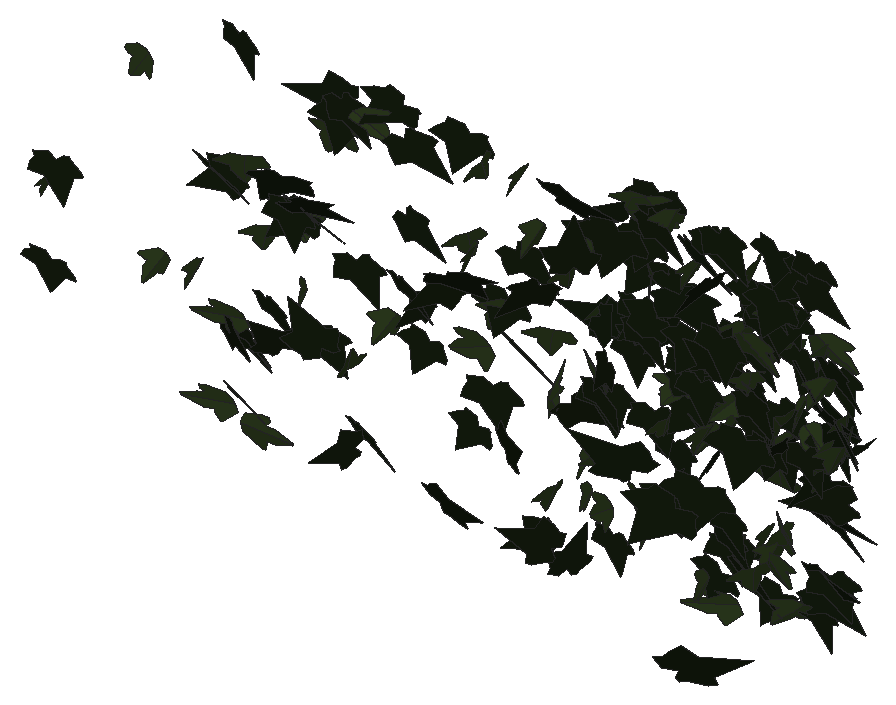
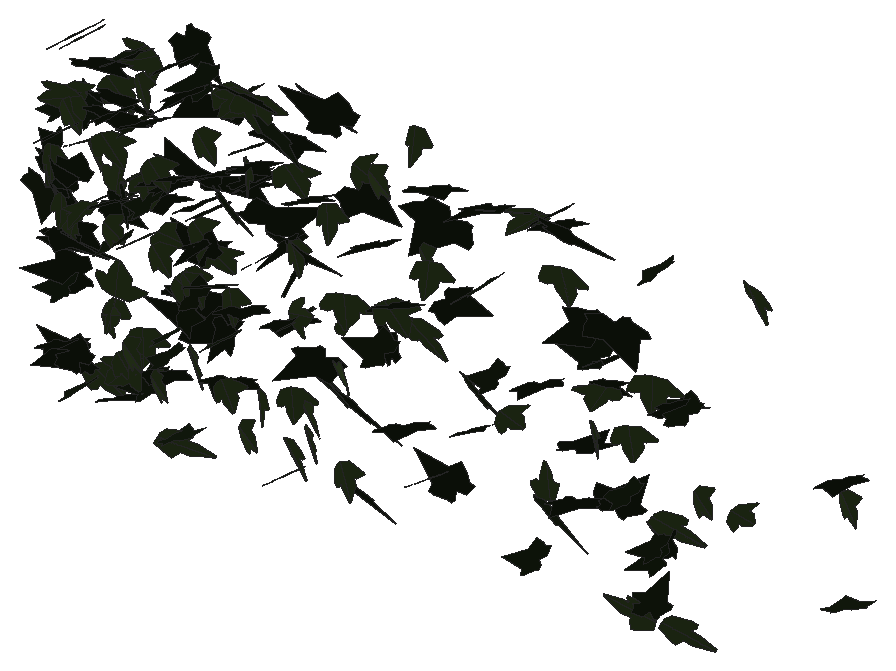
# SketchUp Ruby script. Lengths in millimetres.
U = 1.mm
M = Sketchup.active_model
def pt(a) = Geom::Point3d.new(a.map { |v| v * U })
def face(e, loops, mat)
  f = e.add_face(loops[0].map { |a| pt(a) })
  loops[1..].each { |l| e.add_face(l.map { |a| pt(a) }).erase! }
  f.material = f.back_material = mat if mat
  f
end
# faces: each face lists its corners as indices into pts; further lists are holes
def faces(e, pts, list, mat = nil) = list.each { |f| face(e, (f[0].is_a?(Array) ? f : [f]).map { |l| l.map { |i| pts[i] } }, mat) }
# xy, xz, yz: faces in a plane at the given z, y or x. An outline is a flat list of corners, or four numbers for a rectangle; further outlines are holes
def ring(l) = l.size == 4 ? [[l[0], l[1]], [l[2], l[1]], [l[2], l[3]], [l[0], l[3]]] : l.each_slice(2).to_a
def flat(e, list, mat, &to3) = list.each { |f| face(e, (f[0].is_a?(Array) ? f : [f]).map { |l| ring(l).map { |u, v| to3.(u, v) } }, mat) }
def xy(e, z, list, mat = nil) = flat(e, list, mat) { |x, y| [x, y, z] }
def xz(e, y, list, mat = nil) = flat(e, list, mat) { |x, z| [x, y, z] }
def yz(e, x, list, mat = nil) = flat(e, list, mat) { |y, z| [x, y, z] }
def lines(e, pts, list) = list.each { |a, b| e.add_line(pt(pts[a]), pt(pts[b])) }
# prism: a flat outline (further loops are holes) pulled along v
def prism(e, loops, v, mat = nil)
  f = face(e, loops, mat); d = Geom::Vector3d.new(v.map { |x| x * U })
  f.pushpull(f.normal.samedirection?(d) ? d.length : -d.length)
end
def box(e, o, s, mat = nil) = prism(e, [[o, [o[0] + s[0], o[1], o[2]], [o[0] + s[0], o[1] + s[1], o[2]], [o[0], o[1] + s[1], o[2]]]], [0, 0, s[2]], mat)
def at(x, y, z, deg = 0) = Geom::Transformation.translation(pt([x, y, z])) * Geom::Transformation.rotation(ORIGIN, Z_AXIS, deg.degrees)
def axes(o, x, y, z) = Geom::Transformation.new([*x, 0, *y, 0, *z, 0, *pt(o).to_a, 1])
def part(name) = M.definitions.add(name)
# library, detail: a bought-in or finely detailed component or shape, given as its bounding box
def library(name, o, s) = part(name).tap { |d| box(d.entities, o, s) }
def detail(e, o, s) = box(e.add_group.entities, o, s)
def put(e, d, t, mat = nil) = e.add_instance(d, t).tap { |i| i.material = mat if mat }
def group(e, t, mat = nil) = e.add_group.tap { |g| g.transformation = t; g.material = mat if mat }.entities
root = M.entities
M.materials.add("efeu1").color = [18, 25, 13]
M.materials.add("efeu2").color = [43, 57, 29]
c1 = part("ivyleaf_9")
p = [[39.1,54.8,31.7],[34.5,51.8,30.2],[-5.3,25.2,17.3],[-17.9,28.3,20.9],[-21.6,21.7,17],[-20.2,4.3,5.3],
  [-22.9,-0.3,2.5],[-17.1,-4,-0.6],[-2,-2.1,-1.2],[-0.7,-15.4,-10.1],[16.6,-22.3,-16.7],[21.1,-15.1,-12.5],
  [32.7,-10.7,-11],[46.1,-1.8,-6.6],[30.8,11.2,3.8]]
faces(c1.entities,p,[[0,1,2,3,4,5,6,7,8,9,10,11,12,13,14]],"efeu1")
c2 = part("ivyleaf_10")
p = [[0,12.8,-0.8],[-1.5,51.3,-10.9],[-4.9,51,-11.6],[-13.6,26.5,-7.3],[-13.2,15.9,-4.6],[-21.1,19.3,-7.2],
  [-29.5,16.3,-8.3],[-29.2,8.3,-6.2],[-19.7,-9.8,0.5],[-7.6,-13,4],[1,-12.2,5.8],[-0.4,51.1,-11.1],
  [-1.5,51.1,-10.9],[1,-12.4,5.9],[16.9,-12.4,3.5],[35.1,9.1,-5.1],[35,12.9,-6.1],[20.5,16.4,-4.9],
  [15.8,15,-3.8],[15.3,27.6,-7.1],[12.8,31.3,-7.8]]
faces(c2.entities,p,[[0,1,2,3,4,5,6,7,8,9,10],[11,12,0,13,14,15,16,17,18,19,20]],"efeu2")
put(root,c1,axes([1191.5,726.7,2811.6],[-0.73704,-0.9227,0.38725],[0.48551,-0.49255,-0.91849],[1.84155,-0.23943,0.39714]))
put(root,c2,axes([1219.3,690.7,3035.7],[0.12928,-1.10361,0.0718],[0.0069,-0.07171,-1.1057],[2.10482,0.06802,-0.00078]))
put(root,c1,axes([1236.5,686.2,3073.2],[-0.46682,-1.0606,-0.23525],[0.05512,0.2347,-1.08833],[2.06686,-0.24581,-0.02411]))
put(root,c2,axes([1480.5,663.3,3412.6],[1.55234,-0.77415,-0.31621],[-0.3436,0.26829,-1.1225],[1.55401,0.83264,0.06768]))
put(root,c2,axes([1480.8,715.5,2922.4],[-0.52957,-0.66374,0.83603],[0.24782,-0.87862,-0.65421],[2.01644,-0.06633,0.29997]))
put(root,c2,axes([1568,727.8,2935.1],[0.14688,-1.00594,0.46449],[0.20044,-0.45685,-1.00689],[2.0992,0.11401,0.06364]))
put(root,c2,axes([1619.3,746.9,2625.9],[0.73798,-0.04236,-1.05479],[-1.97272,0.19758,-0.38898],[0.38057,1.1063,0.02908]))
put(root,c1,axes([1568.9,769.3,3147.7],[0.81126,-0.89452,0.54801],[0.73207,-0.41705,-0.97995],[1.85747,0.55505,0.14687]))
put(root,c1,axes([1628.3,774.3,3138.3],[-1.15105,-0.46642,0.84272],[-1.14531,-0.59398,-0.76063],[1.43131,-0.85038,0.06907]))
put(root,c2,axes([1661,727.5,2845.5],[0.75748,0.04113,-1.06387],[-1.98687,0.23796,-0.38136],[0.39763,1.11067,0.1211]))
put(root,c2,axes([1655.3,771.5,3187.5],[-1.73577,-0.69038,-0.05057],[0.0867,0.0236,-1.14383],[1.31459,-0.91312,0.00867]))
put(root,c1,axes([1630.5,785.4,3460.5],[0.32408,-1.0878,0.30446],[0.01875,-0.30645,-1.10045],[2.14978,0.16666,-0.0363]))
put(root,c1,axes([1639,765.1,2786.2],[1.39297,-0.74383,-0.06179],[-0.07632,0.04722,-1.04353],[1.41849,0.73299,0.00453]))
put(root,c1,axes([1637.7,732.2,2818.4],[0.44725,-0.1964,-1.08534],[2.01512,-0.27069,0.27824],[-0.58804,-1.07699,0.12798]))
put(root,c1,axes([1647,761.5,2806],[1.08101,-0.87512,0.10404],[0.12186,-0.08247,-1.04326],[1.67283,0.57153,0.00876]))
put(root,c1,axes([1682.1,744.7,2643.8],[1.3396,-0.90274,0.01591],[-0.01156,0.01544,1.1447],[-1.71832,-0.70388,0.0047]))
put(root,c2,axes([1716.5,767.5,3050.2],[-1.18656,-0.89179,-0.00734],[0.00802,0.00601,-1.08811],[1.6973,-0.62347,0.00001]))
put(root,c2,axes([1713.5,725.8,2609.8],[0.05943,-0.01072,-1.17609],[2.03876,-0.48546,0.03287],[-0.92414,-1.07168,-0.00312]))
put(root,c1,axes([1730.4,753.2,2894.1],[0.82906,-0.99043,0.25411],[0.24944,-0.21985,-1.08156],[1.92998,0.45387,0.03063]))
put(root,c1,axes([1794.5,715.4,2829.2],[0.83202,0.15121,1.08821],[-1.90885,-0.42313,0.46172],[0.85349,-1.09374,-0.02818]))
put(root,c1,axes([1814.4,692.6,3235.3],[1.02406,0.6933,-0.78828],[-0.91417,-0.62504,-0.8776],[-1.77654,0.72127,-0.0028]))
put(root,c1,axes([1818.3,761.1,3122.2],[-1.43198,-0.6843,0.4398],[-0.6418,-0.28278,-1.01692],[1.40885,-0.82436,-0.01624]))
put(root,c2,axes([1792.2,758.6,3117.1],[1.31541,0.81659,0.26113],[0.31065,0.20395,-1.0698],[-1.60181,0.71014,0.00697]))
put(root,c1,axes([1822.3,710.1,3159.6],[-0.38177,-1.13323,0.06662],[0.02718,-0.07017,-1.15055],[2.16032,-0.19938,0.02625]))
put(root,c2,axes([1860,705.7,2983.8],[0.51658,-0.85202,-0.61381],[-0.23458,0.60376,-0.89256],[1.98474,0.29312,0.05427]))
put(root,c1,axes([1849.3,774.5,2850.7],[-0.18895,-0.9378,-0.60059],[0.35882,0.58011,-0.93699],[2.08887,-0.18448,0.10663]))
put(root,c1,axes([1837.3,719.4,3164.6],[1.07616,-0.74923,0.57769],[0.87104,-0.3724,-0.93094],[1.57587,0.71748,0.12006]))
put(root,c2,axes([1904.8,755.4,3345],[-2.0098,0.10997,0.37654],[-0.72813,-0.04991,-1.05838],[-0.16488,-1.12002,0.08413]))
put(root,c1,axes([1934,744.2,3435.5],[-1.46269,0.43127,0.72687],[-1.31073,0.24993,-0.87647],[-0.93241,-1.02787,0.09185]))
put(root,c1,axes([1861.4,678.6,3198.7],[1.91747,0.36353,0.53751],[0.93447,0.22194,-1.07042],[-0.80745,1.12014,0.03765]))
put(root,c1,axes([1931,669.2,2897.8],[-1.70733,-0.79083,0.33482],[0.48594,0.21668,1.19588],[-1.56053,0.93269,0.00608]))
put(root,c2,axes([1948.8,744.8,2822.7],[-0.23159,-1.0582,-0.41002],[-0.09822,-0.40678,1.06516],[-2.15763,0.1321,-0.00448]))
put(root,c1,axes([1958.1,714.2,3425.6],[-0.97639,-1.02415,0.01667],[-0.01341,-0.01512,-1.14546],[1.94938,-0.51307,0.00047]))
put(root,c1,axes([1955.1,713.8,3452.1],[0.46753,-1.06693,-0.34846],[-0.02372,0.35409,-1.09296],[2.136,0.23746,0.06413]))
put(root,c1,axes([1965.9,748.6,3068.4],[-0.15212,-1.07471,-0.41201],[0.1907,0.40493,-1.0757],[2.18222,-0.1103,0.06528]))
put(root,c1,axes([1955.6,767.2,2675.1],[1.0953,-0.91051,0.29425],[0.28784,-0.2525,-1.07712],[1.79824,0.59501,-0.00681]))
put(root,c1,axes([2042.7,637.9,2715.3],[-1.74553,0.88546,-0.13495],[0.16492,-0.10452,-1.27475],[-1.69667,-0.92112,0.01492]))
put(root,c2,axes([2001.6,717.6,3429],[0.76985,0.81164,0.72364],[0.63449,0.64234,-0.90681],[-1.96986,0.5241,-0.00927]))
put(root,c1,axes([2054.2,779.1,3451.1],[-1.8053,-0.49486,0.40687],[-0.26601,-0.54959,-0.99429],[1.18991,-0.87365,0.39501]))
put(root,c2,axes([2049.2,750.7,2966.4],[-0.59425,-0.75686,0.82967],[0.20286,-0.87723,-0.76012],[2.1277,-0.12775,0.30419]))
put(root,c1,axes([2064.7,765,3052.5],[0.94934,-0.93714,0.27791],[0.23988,-0.24773,-1.06161],[1.8448,0.51446,-0.00497]))
put(root,c1,axes([2126.8,771.1,3021.4],[-1.68606,0.51029,-0.44101],[0.67101,-0.27026,-1.02096],[-1.09426,-0.95199,0.05345]))
put(root,c1,axes([2118.4,784.8,2922.4],[-0.82895,-0.90485,0.38544],[-0.14646,-0.3889,-0.99993],[1.86609,-0.43247,0.09274]))
put(root,c1,axes([2118.6,722.6,3236.6],[0.94969,-0.95515,-0.51361],[-0.23035,0.51279,-1.07121],[2.05109,0.49984,0.11751]))
put(root,c1,axes([2113.3,722.9,3414.7],[0.49617,-0.89498,-0.76674],[0.38231,0.80754,-0.87429],[2.21012,0.06123,0.32337]))
put(root,c1,axes([2228.8,778.2,3442.4],[-1.31551,-0.91987,0.0399],[0.09443,-0.08703,-1.14695],[1.7498,-0.68687,0.09189]))
put(root,c1,axes([2246.9,691.6,3138.7],[-0.22712,0.03025,-1.214],[0.40279,-1.20066,-0.05073],[-2.27583,-0.21552,0.11218]))
put(root,c1,axes([2239.1,793.1,2765.5],[-0.84301,-0.72773,0.60696],[-0.3205,-0.59888,-0.84094],[1.77481,-0.45381,0.13644]))
put(root,c2,axes([2252.6,745.4,3231.4],[-0.97311,-1.01793,-0.36269],[0.29064,0.32915,-1.13908],[2.03599,-0.53351,-0.01075]))
put(root,c2,axes([2294.7,706.2,3232.2],[0.4884,-1.08207,0.21063],[0.11421,-0.20223,-1.11202],[2.09494,0.26329,0.01152]))
put(root,c1,axes([2285.2,784.9,2874.5],[-0.61366,-1.11278,-0.29915],[0.24553,0.27382,-1.15764],[2.17926,-0.3442,0.04619]))
put(root,c2,axes([2338.6,677.8,3037.5],[1.42315,-0.37964,-0.89561],[-1.4218,0.49937,-0.83542],[1.18571,1.05446,0.07319]))
put(root,c1,axes([2274.4,637.2,2668.1],[0.29322,-0.39236,1.1611],[1.24044,-0.96482,-0.41251],[1.97539,0.66409,0.08669]))
put(root,c2,axes([2354.3,745.8,3104.6],[-1.04631,-0.95739,0.43782],[-0.32281,-0.40692,-1.1028],[1.97742,-0.57301,0.05164]))
put(root,c2,axes([2352.4,662.9,3471.5],[-0.24852,-1.05676,-0.63879],[0.2446,0.62724,-1.06391],[2.33736,-0.178,0.04342]))
put(root,c1,axes([2350.4,752.3,3115],[-1.06347,-0.95758,0.09599],[-0.05881,-0.09309,-1.10851],[1.83066,-0.55927,0.02015]))
put(root,c1,axes([2337.3,576.5,3241.5],[2.07846,0.78995,0.16363],[0.25049,0.09724,-1.34784],[-1.51478,1.09999,0.00164]))
put(root,c2,axes([2372.5,770.8,3414.6],[0.37614,-1.02003,0.48855],[0.12434,-0.48482,-1.03869],[2.1489,0.2066,-0.02541]))
put(root,c1,axes([2356.2,766.1,3010.1],[0.99279,-0.91056,0.61644],[0.70797,-0.49593,-1.04734],[1.96938,0.63731,0.06575]))
put(root,c1,axes([2386.7,741.6,3243.5],[0.51282,-0.9044,-0.61716],[0.26464,0.65869,-0.90456],[2.06696,0.14005,0.26893]))
put(root,c2,axes([2452.5,770.3,2706.2],[-0.24645,-1.19814,-0.09629],[0.02746,0.09529,-1.20511],[2.28748,-0.13023,0.00409]))
put(root,c1,axes([2486.4,711.7,2636],[-1.9791,0.40389,0.05562],[-0.10392,0.01304,-1.11554],[-0.76895,-1.04129,0.00761]))
put(root,c2,axes([2471.3,747.1,3081.4],[-1.70009,-0.63308,0.04333],[-0.06927,-0.02357,-1.09487],[1.2057,-0.89402,-0.00181]))
put(root,c2,axes([2446.5,777.3,2915.6],[-0.3315,-0.2576,-1.08193],[0.57785,-1.06454,0.20458],[-2.03629,-0.26015,0.23419]))
put(root,c2,axes([2483.4,681.9,3356.3],[-0.15927,-0.86997,0.8758],[0.37,-0.87614,-0.85174],[2.32009,0.08,0.19595]))
put(root,c1,axes([2478.1,588,2886.7],[-0.03405,0.07483,1.28295],[0.28258,-1.27436,0.0764],[2.42948,0.14927,0.00909]))
put(root,c1,axes([2528.8,625.5,3262.8],[-0.18308,0.58477,-1.146],[0.1864,-1.14254,-0.59122],[-2.44151,-0.13108,0.0408]))
put(root,c2,axes([2527.1,728.6,3259.4],[-0.38862,-1.14307,-0.35777],[0.11778,0.35238,-1.16117],[2.27652,-0.21336,-0.001]))
put(root,c2,axes([2519.4,690.2,2992.3],[0.88527,-1.08626,0.44322],[-0.33888,0.4059,1.18165],[-2.20697,-0.49805,-0.00366]))
put(root,c1,axes([2546.9,795.4,3308.6],[-1.33942,-0.678,0.57243],[-0.50237,-0.53758,-0.96124],[1.61232,-0.73074,0.17604]))
put(root,c2,axes([2538.1,776.9,2811.9],[0.8656,-0.96083,0.18533],[0.09872,-0.18041,-1.06262],[1.85974,0.45679,-0.02985]))
put(root,c1,axes([2522.1,752.1,2933.8],[0.04894,-0.09389,-1.23097],[0.05146,1.23098,-0.09333],[2.34902,-0.02501,0.02769]))
put(root,c2,axes([2558.4,750.7,2742.9],[0.81548,-0.938,-0.19948],[-0.06794,0.20274,-1.02998],[1.82386,0.42695,0.05082]))
put(root,c1,axes([2609.6,560.4,2717.8],[-1.30625,0.81521,0.76926],[-1.02719,0.5502,-1.06461],[-1.86964,-0.87185,0.04745]))
put(root,c2,axes([2593.7,749.9,3009.7],[-0.56238,0.55739,-1.02446],[-1.00581,0.87811,0.63019],[1.9787,0.60478,0.02917]))
put(root,c2,axes([2582.4,767.6,3173.6],[-0.06665,-1.08991,-0.11285],[0.04084,0.11221,-1.09032],[2.085,-0.03704,0.01775]))
put(root,c2,axes([2593.4,766.4,2711.5],[1.05003,-0.79291,-0.71078],[-0.72246,0.60148,-0.96563],[1.89348,0.6692,0.02573]))
put(root,c2,axes([2590.9,773.4,3349.8],[-1.21151,-0.83611,0.45098],[-0.24202,-0.46298,-1.03786],[1.79172,-0.62789,0.16474]))
put(root,c1,axes([2623.7,749.9,3158.3],[-1.10622,0.53675,0.84229],[-1.39906,0.42982,-0.78119],[-1.28682,-0.92873,0.12525]))
put(root,c2,axes([2589.4,764,2830.1],[-0.86451,-0.97776,-0.16181],[0.07595,0.15981,-1.07768],[1.88466,-0.45495,-0.03079]))
put(root,c1,axes([2536.6,688.2,3445.9],[0.70627,-0.5199,1.09019],[1.70784,-0.6447,-0.6129],[1.53863,0.95425,0.17988]))
put(root,c1,axes([2591.1,745.5,2997.5],[0.36691,-1.09365,0.0702],[0.02103,-0.06933,-1.11051],[2.08561,0.1931,-0.00115]))
put(root,c1,axes([2601.8,778.7,2644.8],[-0.10704,-1.02992,0.14554],[0.02246,-0.14638,-1.03127],[1.9795,-0.05403,0.01957]))
put(root,c1,axes([2604.5,757.7,2993.4],[-0.57026,-1.1328,-0.24164],[0.14129,0.2303,-1.17169],[2.19993,-0.30844,0.01261]))
put(root,c1,axes([2607.2,736.6,3171.1],[0.82022,-0.44761,-1.03942],[-0.75517,0.98187,-0.58734],[2.01713,0.5496,0.20277]))
put(root,c1,axes([2654.2,757.3,3423.8],[-0.77575,1.02057,0.29385],[-0.40326,0.23028,-1.09368],[-1.98062,-0.44661,0.10758]))
put(root,c1,axes([2620,733.8,3071.4],[0.34521,-0.41129,-1.06261],[1.34342,-0.8041,0.43172],[-1.70233,-0.71797,0.12521]))
put(root,c1,axes([2663.1,573.3,3385],[-2.11644,0.71545,-0.1428],[-0.22795,0.07776,1.32231],[1.36966,1.11847,-0.00059]))
put(root,c1,axes([2656.9,723.8,3390.1],[-1.95209,-0.68214,-0.36904],[0.54568,0.23503,-1.2313],[1.37149,-1.06442,-0.03537]))
put(root,c2,axes([2694.8,758.3,3466.7],[-1.78426,-0.63695,0.15688],[-0.23547,-0.09704,-1.13336],[1.22606,-0.94558,0.01063]))
put(root,c2,axes([2686,745.8,2782.8],[0.90791,-0.75654,-0.5686],[-0.05408,0.62501,-0.85544],[1.80035,0.40029,0.26104]))
put(root,c1,axes([2670.9,761.1,3115.5],[-0.15858,-1.07629,0.25389],[-0.07473,-0.25157,-1.07934],[2.10328,-0.09009,-0.01921]))
put(root,c1,axes([2692.1,519.6,2720.9],[-1.51181,1.04419,-0.28104],[-0.34163,0.21655,1.31195],[2.02948,0.8143,0.01149]))
put(root,c1,axes([2694.2,774.7,3371.2],[-0.77844,-0.97551,0.44923],[-0.14323,-0.45349,-1.05328],[2.03896,-0.40429,0.09752]))
put(root,c1,axes([2708.7,768.4,3319],[-1.23066,-0.87397,0.31345],[-0.33958,-0.25789,-1.08713],[1.73414,-0.67073,0.00956]))
put(root,c2,axes([2701.3,779.2,2710.9],[0.46306,-0.95253,0.5263],[0.29177,-0.50391,-0.98289],[2.05052,0.28681,0.02101]))
put(root,c2,axes([2723.2,744.2,3303.8],[0.87341,-0.922,-0.44073],[0.08541,0.50084,-1.00103],[1.94304,0.39243,0.24211]))
put(root,c2,axes([2717.1,757.3,3467.6],[-1.78354,-0.3643,-0.56454],[1.0307,0.16389,-1.00473],[0.75683,-1.08169,0.0379]))
put(root,c1,axes([2724.2,771,3482.9],[-1.65371,-0.55862,-0.51625],[1.11045,0.01334,-0.99648],[0.92876,-1.01061,0.2722]))
put(root,c1,axes([2723.7,760.7,2980.9],[-0.49655,-0.99125,-0.37424],[0.23751,0.35399,-1.02461],[2.00249,-0.28778,0.02873]))
put(root,c1,axes([2723.1,711.7,3254.2],[0.00599,-1.149,-0.06359],[-0.00471,0.06358,-1.149],[2.19011,0.00328,-0.0023]))
put(root,c2,axes([2752.8,778.6,2798.3],[-0.48958,-1.02638,0.14823],[0.02003,-0.1553,-1.05706],[1.97358,-0.25304,0.0475]))
put(root,c1,axes([2766.2,705.7,3240],[-1.02933,-0.75527,0.7338],[-0.8138,-0.59635,-0.92895],[1.8315,-0.68946,-0.00036]))
put(root,c2,axes([2766.4,740.9,2985.8],[-0.28316,-1.07995,-0.24936],[0.06937,0.2467,-1.09015],[2.1083,-0.15316,0.00238]))
put(root,c1,axes([2741.2,723.1,3454.7],[0.84207,-1.02896,-0.33743],[-0.11316,0.34087,-1.11743],[2.05781,0.4398,0.07663]))
put(root,c1,axes([2754.2,760.2,2805.3],[-0.69403,-0.88392,-0.53568],[0.40922,0.49074,-0.95613],[1.92405,-0.42321,0.01013]))
put(root,c2,axes([2774.4,754.3,3460.8],[-0.60065,-1.0866,0.26717],[0.12653,-0.29532,-1.12252],[2.12584,-0.28944,0.1423]))
put(root,c1,axes([2787.5,748,3208.3],[-1.63472,0.55562,-0.45715],[0.69657,-0.27552,-1.02254],[-1.17897,-0.93319,0.02972]))
put(root,c1,axes([2750.8,678.6,3230.4],[0.40103,-1.07809,-0.24271],[0.00626,0.2477,-1.09737],[2.10317,0.20483,0.04955]))
put(root,c1,axes([2754.7,787,2907.6],[0.09371,-1.09588,0.10407],[0.05113,-0.10294,-1.09677],[2.09444,0.05155,0.02212]))
put(root,c1,axes([2775.3,785.8,3286.8],[-0.91398,-0.96745,0.34109],[-0.10943,-0.35064,-1.07548],[1.94926,-0.47331,0.09956]))
put(root,c2,axes([2800.1,756.6,3078.5],[-1.2547,-0.60403,0.65453],[-0.28539,-0.72743,-0.82234],[1.67089,-0.57782,0.35104]))
put(root,c1,axes([2810,786,3014.4],[-1.38378,-0.74656,0.38538],[-0.13545,-0.45309,-1.01201],[1.59325,-0.68693,0.24867]))
put(root,c2,axes([2816.1,775.3,3349.2],[-0.07727,-1.10928,0.31414],[-0.00883,-0.31417,-1.11],[2.19419,-0.04033,0.00659]))
put(root,c1,axes([2822.9,687.4,2872],[-0.1251,0.22427,-1.26075],[-1.46511,1.00191,0.21836],[1.94757,0.76811,0.08329]))
put(root,c1,axes([2861.7,502.6,3015.8],[0.30491,0.13331,1.3584],[-2.59179,-0.07688,0.16816],[0.17567,-1.36566,0.12313]))
put(root,c1,axes([2809.8,760.2,3100],[0.18421,-0.82078,-0.76965],[0.0831,0.77465,-0.82062],[2.13985,0.04057,0.09812]))
put(root,c2,axes([2837.9,758.7,3127.5],[-0.34587,-0.97374,0.46335],[0.03992,-0.47299,-0.98577],[2.05195,-0.15493,0.09728]))
put(root,c1,axes([2814.5,768.2,3077.5],[0.24193,-0.40458,1.03959],[1.042,-0.889,-0.41292],[1.8498,0.55369,0.09664]))
put(root,c1,axes([2832.6,728.9,3157.7],[0.00239,-1.11665,-0.03964],[0.01373,0.03965,-1.11663],[2.1265,0.001,0.00726]))
put(root,c1,axes([2824.5,779.6,2980.7],[0.85104,-0.83404,0.51296],[0.48241,-0.4461,-0.94628],[1.80001,0.51389,0.01108]))
put(root,c2,axes([2866.9,745.6,2996.1],[-0.17736,-1.22064,0.12956],[-0.03714,-0.12845,-1.22416],[2.33588,-0.09472,-0.00963]))
put(root,c1,axes([2867.4,716.4,3216.1],[-1.13683,-0.89897,0.39954],[-0.15147,-0.42173,-1.06789],[1.86615,-0.58187,0.15671]))
put(root,c2,axes([2874.3,767.5,2990.3],[-0.2987,-0.89912,0.64092],[-0.02442,-0.64583,-0.90916],[2.10132,-0.13532,0.08054]))
put(root,c1,axes([2864.8,795.8,2645.1],[-0.82177,-0.78665,0.66719],[0.03883,-0.72966,-0.84711],[1.96275,-0.31493,0.2961]))
put(root,c1,axes([2872.2,770.2,2926.9],[-0.75737,0.01975,-1.03994],[1.3082,-0.83067,-0.2788],[-1.48571,-0.7415,0.28464]))
put(root,c2,axes([2914.8,754.5,2607.4],[0.64445,0.08867,-1.07915],[-2.00608,-0.23175,-0.34978],[-0.47158,1.10703,0.01321]))
put(root,c1,axes([2861.5,767.1,3436.3],[0.28772,-1.04498,-0.44736],[-0.04073,0.4486,-1.05511],[2.163,0.14745,0.03964]))
put(root,c1,axes([2853.1,709.6,3439.3],[1.53342,-0.96704,0.02435],[0.0307,-0.01825,-1.2587],[1.84079,0.80587,0.00071]))
put(root,c1,axes([2893.2,697.4,3135.3],[-0.30875,-1.09652,0.09856],[-0.00184,-0.09948,-1.10837],[2.09531,-0.16166,0.01355]))
put(root,c1,axes([2879.9,650.8,3353.5],[-0.53699,-0.65621,-1.04476],[1.3315,0.79766,-0.68994],[1.93404,-0.73135,0.18491]))
put(root,c2,axes([2930.9,755,3079.3],[0.52663,0.65594,-0.85393],[-1.05311,-0.66974,-0.69376],[-1.75805,0.59768,0.15978]))
put(root,c1,axes([2917.7,673.2,2910.9],[-1.81295,-0.80439,-0.37029],[0.54855,0.2326,-1.24675],[1.59356,-0.9952,0.0079]))
put(root,c2,axes([2926.4,779.8,3048.4],[-0.16702,-1.04924,0.33224],[0.04508,-0.33502,-1.05175],[2.09414,-0.07647,0.04914]))
put(root,c1,axes([2917.4,683.2,3190.2],[-1.77753,0.54075,0.74765],[1.22308,-0.38215,1.07919],[1.26014,1.13368,0.00716]))
put(root,c1,axes([2926.3,784.6,3216.8],[-1.01277,-0.94889,0.25723],[-0.13404,-0.25495,-1.08618],[1.8663,-0.53324,0.06158]))
put(root,c2,axes([2935,781.9,3244.6],[-0.56392,-1.01829,0.39619],[-0.0562,-0.40289,-1.05759],[2.07878,-0.28713,0.07888]))
put(root,c2,axes([2928.8,781.5,2748.7],[0.55551,-0.92671,0.45216],[0.25162,-0.43242,-0.97158],[1.94625,0.32041,-0.00345]))
put(root,c1,axes([2917.4,736.1,3193.8],[0.16847,-1.01238,-0.52262],[-0.07918,0.52097,-1.01624],[2.16691,0.09775,0.0035]))
put(root,c1,axes([2916,732,3470.2],[0.35246,-1.16517,-0.30096],[0.0482,0.30821,-1.17765],[2.28983,0.17286,0.07111]))
put(root,c1,axes([2933.9,753,2756],[-0.7297,-0.91126,-0.40207],[0.27097,0.37626,-0.98853],[1.87615,-0.40876,-0.0136]))
put(root,c2,axes([2954.9,628.9,2731.1],[0.92162,-1.06011,-0.21104],[-0.09644,0.20873,-1.16479],[2.05493,0.48525,0.03998]))
put(root,c1,axes([2934.3,727.5,2833.6],[0.33311,-1.07468,0.03545],[0.01791,-0.03439,-1.08884],[2.04637,0.17524,0.00376]))
put(root,c1,axes([2930.8,738.3,2784],[0.53499,-1.02226,0.22096],[0.14423,-0.20829,-1.06006],[1.98527,0.29061,0.01747]))
put(root,c1,axes([2987.6,606.4,3445.8],[-0.73094,0.96601,-0.88686],[0.64617,-0.81936,-1.03951],[-2.41071,-0.51252,-0.00973]))
put(root,c2,axes([2979.7,767,3417.1],[0.17853,-1.14469,-0.13274],[0.00148,0.13324,-1.14846],[2.19316,0.09309,0.01158]))
put(root,c1,axes([2972.1,787.8,3334.2],[-0.93041,-0.96241,0.31879],[-0.10165,-0.32897,-1.07507],[1.92684,-0.48207,0.09722]))
put(root,c2,axes([2991.1,733.3,3172.2],[-1.11242,-0.96213,-0.024],[0.02118,0.02132,-1.12576],[1.83158,-0.5846,-0.00156]))
put(root,c1,axes([2957,767.6,3146.3],[0.84477,-0.99292,0.21512],[0.12521,-0.20617,-1.08736],[1.92951,0.44809,-0.02362]))
put(root,c1,axes([2964.3,768.8,3220.6],[0.52057,-1.10581,-0.19013],[-0.07637,0.18593,-1.13912],[2.13409,0.27639,0.00562]))
put(root,c1,axes([2964.5,741.5,2717.7],[1.30817,-1.06043,0.13032],[0.13488,-0.10937,-1.26371],[2.02892,0.69099,-0.00001]))
put(root,c2,axes([3001.6,778.9,2799],[0.4157,-1.05759,0.41737],[0.14271,-0.41068,-1.07988],[2.15917,0.23076,-0.00898]))
put(root,c1,axes([3004.2,759.6,3037.2],[-0.71499,-0.84617,0.61729],[-0.26871,-0.6089,-0.92059],[1.97523,-0.38913,0.09821]))
put(root,c2,axes([3019.6,777.7,2767.1],[-0.38112,-0.98394,0.3749],[0.05903,-0.38696,-0.99904],[2.00308,-0.17581,0.10077]))
put(root,c1,axes([3000.8,632.2,3302.7],[-0.29962,-1.23369,0.2559],[-0.04013,-0.25528,-1.24364],[2.3976,-0.15844,0.01116]))
put(root,c1,axes([3038.5,424.2,3017.5],[-2.1039,-0.855,0.27966],[-0.42852,-0.16598,-1.3975],[1.65757,-1.12813,-0.00633]))
put(root,c1,axes([3001.9,750,3306.3],[0.44176,-1.09957,0.10858],[0.02116,-0.10862,-1.12374],[2.10277,0.2321,-0.0115]))
put(root,c2,axes([3015.7,769.4,2743.2],[-1.78977,0.436,-0.41275],[0.68521,-0.20429,-1.03608],[-0.9144,-1.00647,0.0315]))
put(root,c2,axes([3033,776.6,2925.2],[-2.12799,0.08461,0.04764],[0.08284,-0.05549,1.1201],[0.16519,1.11775,0.05201]))
put(root,c1,axes([3013.4,702.2,3140],[0.62171,-1.06419,-0.17164],[-0.0789,0.16682,-1.11316],[2.05003,0.32916,0.00921]))
put(root,c1,axes([3042.1,769.4,2668],[-1.09181,-0.83343,0.32274],[-0.10879,-0.3485,-1.00157],[1.69748,-0.5584,0.14339]))
put(root,c1,axes([3030.8,773.3,3456.6],[-0.45103,-0.98415,0.52069],[-0.04198,-0.5281,-1.00819],[2.11861,-0.21998,0.09087]))
put(root,c2,axes([3046.5,674.6,2766.8],[-0.90959,-1.09363,-0.23784],[0.16285,0.22216,-1.19346],[2.12382,-0.48542,-0.01035]))
put(root,c1,axes([3076.6,762.8,3353.6],[-2.03798,-0.1366,0.39034],[-0.71895,-0.11783,-1.07754],[0.32031,-1.13364,0.06496]))
put(root,c2,axes([3062,776.1,3258.2],[-0.956,-0.92838,0.38137],[-0.37231,-0.32772,-1.05545],[1.87353,-0.53885,-0.01514]))
put(root,c1,axes([3045.5,651.2,3073.8],[-1.21438,-1.16576,0.00062],[0.00673,-0.00265,-1.32895],[2.21867,-0.63807,0.00437]))
put(root,c1,axes([3038.5,783.4,3333.1],[0.01389,-1.11482,-0.15801],[0.0387,0.15812,-1.11464],[2.14258,0.00437,0.02115]))
put(root,c1,axes([3054.4,767.5,3323.1],[-1.58663,-0.67955,-0.38777],[0.73363,0.13637,-1.06769],[1.29581,-0.90927,0.12968]))
put(root,c2,axes([3070.7,754,3045.8],[0.08519,-0.90283,0.65318],[0.2331,-0.64576,-0.90097],[2.10796,0.1079,0.07323]))
put(root,c2,axes([3086.2,721.7,3356],[-0.77108,-1.07486,0.48397],[-0.28165,-0.46133,-1.14847],[2.22573,-0.43075,0.02234]))
put(root,c1,axes([3055.7,759,3011.7],[0.05734,-1.0575,0.33625],[0.07935,-0.33506,-1.05749],[2.11044,0.04133,0.03062]))
put(root,c2,axes([3096.1,728.9,2821.1],[-0.59328,0.61857,-0.93908],[-0.77154,0.84714,0.69258],[1.99623,0.51126,-0.01141]))
put(root,c1,axes([3065.3,701.2,3042.6],[-0.4136,-0.89513,0.63774],[0.03419,-0.6529,-0.91027],[2.09148,-0.16634,0.141]))
put(root,c2,axes([3079,725.8,2846.8],[-0.37851,-0.90444,-0.56599],[0.3821,0.53373,-0.92343],[1.99432,-0.27392,0.06951]))
put(root,c1,axes([3055.8,754.6,3112],[0.48306,-0.99051,-0.46726],[0.30115,0.50778,-0.99045],[2.06249,0.15785,0.25405]))
put(root,c1,axes([3075.7,706.4,3090.8],[-0.8205,0.29112,-1.14791],[1.76746,-0.67493,-0.51995],[-1.39858,-1.02374,0.01635]))
put(root,c1,axes([3102.8,774.3,3426.5],[-1.80929,-0.6272,0.21778],[-0.27309,-0.17728,-1.1369],[1.23374,-0.95904,0.06773]))
put(root,c1,axes([3105.7,704.3,3070.1],[-0.82428,0.45574,-0.93139],[0.65589,-0.88872,-0.59511],[-1.86126,-0.51501,0.20276]))
put(root,c2,axes([3116.5,729.4,2683.1],[-0.97005,-0.76914,0.62804],[-0.66049,-0.52344,-0.92269],[1.77066,-0.61663,-0.00011]))
put(root,c1,axes([3097.7,686.4,3401.2],[-0.89386,-0.98914,0.37014],[-0.15866,-0.3691,-1.09215],[2.00374,-0.47047,0.07864]))
put(root,c2,axes([3100.9,699.1,3112.3],[-0.21539,-0.84043,-0.93885],[-0.14145,-0.93654,0.84732],[-2.39398,0.13095,0.03441]))
put(root,c1,axes([3068.3,415.9,2659.2],[0.27518,-0.08116,1.41192],[2.67342,0.17295,-0.13391],[-0.31237,1.40873,0.09778]))
put(root,c1,axes([3119.8,769.7,3233.9],[-0.80414,-0.9618,0.39733],[0.04094,-0.43681,-1.03449],[1.98011,-0.38156,0.18275]))
put(root,c2,axes([3104,589.5,3355.3],[-1.48973,0.49504,-0.82855],[1.31065,-0.46098,-0.92602],[-1.28704,-1.04244,0.01603]))
put(root,c2,axes([3126,760.1,3076.6],[0.43126,1.03358,0.42909],[0.17066,0.41962,-1.05812],[-2.12304,0.24369,0.0021]))
put(root,c1,axes([3126.1,779.9,2664.5],[0.25447,-1.13293,0.15237],[-0.01036,-0.15404,-1.14056],[2.17558,0.13178,-0.02325]))
put(root,c2,axes([3148.7,705.6,3174.8],[0.78931,-1.03962,0.30394],[0.26234,-0.27215,-1.11898],[2.04467,0.43624,0.02624]))
put(root,c1,axes([3135.8,761.8,3465.3],[-0.08295,-1.14776,0.22142],[-0.02649,-0.22105,-1.14858],[2.22454,-0.04543,-0.00542]))
put(root,c1,axes([3150,716.5,3057.7],[0.10356,-1.11069,-0.05596],[0.00054,0.05604,-1.11202],[2.11655,0.05433,0.00302]))
put(root,c2,axes([3173.9,759.1,3289.3],[-0.06666,-1.11742,0.22972],[-0.00052,-0.22982,-1.11795],[2.17116,-0.03436,0.00678]))
put(root,c1,axes([3132.9,781.2,2727.2],[0.48932,-0.38242,1.05071],[1.12605,-0.8683,-0.4608],[1.80571,0.6451,0.00263]))
put(root,c1,axes([3189.2,740.8,2991.7],[0.07994,0.35924,-1.0748],[-0.11357,-1.07335,-0.36108],[-2.15381,0.06993,-0.02085]))
put(root,c2,axes([3178.5,743.9,3001.8],[-0.43239,-0.68738,-0.8885],[-0.3011,-0.87788,0.71962],[-2.11667,0.2653,0.07913]))
put(root,c2,axes([3183.5,764.8,3072.1],[-0.42435,-1.02658,-0.33738],[0.27715,0.3128,-1.04803],[2.03783,-0.25631,0.07228]))
put(root,c1,axes([3172.1,771.4,2750.4],[-0.30885,-0.99267,-0.47818],[0.25171,0.46229,-1.00458],[2.08186,-0.20316,0.05052]))
put(root,c1,axes([3165.5,707,3452],[0.95186,-0.85881,-0.64286],[-0.21759,0.66258,-0.9741],[2.03005,0.4737,0.19702]))
put(root,c1,axes([3158.9,760.7,2713.8],[-0.20869,-0.53448,-0.92771],[1.23058,0.71024,-0.48561],[1.62413,-0.60682,0.24874]))
put(root,c1,axes([3148,751.6,2911],[1.80813,-0.32352,0.53916],[0.9636,-0.18567,-1.00356],[0.7096,1.07648,-0.01106]))
put(root,c1,axes([3153.3,760.5,3131.6],[0.53368,-0.58159,0.91123],[1.10152,-0.71432,-0.63402],[1.73766,0.63144,0.12205]))
put(root,c1,axes([3232.3,738.3,2957.9],[-1.72253,-0.05997,0.71402],[-1.35551,-0.05071,-0.90705],[0.14938,-1.1517,0.00275]))
put(root,c1,axes([3171.3,691.8,3237.3],[-0.05516,-0.47694,1.18997],[0.17349,-1.18803,-0.47394],[2.43371,0.07388,0.06076]))
put(root,c1,axes([3164.7,776.5,2885.7],[1.10646,-0.89238,0.22109],[0.19054,-0.19858,-1.06478],[1.73933,0.58944,-0.024]))
put(root,c1,axes([3227.8,749.5,3108.7],[0.02586,-0.08953,1.1406],[-0.81969,1.05637,0.08805],[-2.01728,-0.43039,-0.02116]))
put(root,c2,axes([3174.7,749.3,3307.9],[-1.51213,0.06631,-0.84981],[1.49539,-0.39343,-0.7653],[-0.62895,-1.09483,0.22355]))
put(root,c1,axes([3189.5,771.7,3231.8],[0.0422,-1.12343,-0.05151],[0.00614,0.05158,-1.12364],[2.14036,0.022,0.00424]))
put(root,c1,axes([3188.8,757.3,3100.5],[-0.70501,0.05683,-1.14627],[2.15274,-0.1858,-0.37475],[-0.36972,-1.19022,0.00377]))
put(root,c2,axes([3233.4,673,3264.1],[-0.45015,-0.95803,0.59751],[0.00464,-0.61091,-0.97855],[2.14887,-0.19937,0.12728]))
put(root,c2,axes([3230.4,741.7,3156.9],[-0.24091,-1.03452,-0.43706],[0.13965,0.43127,-1.04207],[2.13284,-0.14509,0.01886]))
put(root,c1,axes([3202.6,729.1,3269.3],[0.9284,-1.02484,0.12803],[0.07003,-0.12425,-1.13483],[1.96438,0.48878,-0.02005]))
put(root,c2,axes([3239.9,708.2,3095.9],[-0.6981,-1.04887,0.15004],[-0.05981,-0.14794,-1.11099],[2.01563,-0.36766,0.019]))
put(root,c1,axes([3245.4,746.5,3071.9],[0.24225,0.99317,0.60816],[0.10567,0.60591,-1.00112],[-2.21391,0.13759,0.01876]))
put(root,c2,axes([3230.2,752.8,3115.3],[0.95425,-0.90225,0.51215],[0.56161,-0.4213,-1.0311],[1.89297,0.57982,0.04774]))
put(root,c1,axes([3252,704.6,3140.5],[0.84168,-0.21275,-1.09936],[1.82539,-0.53804,0.48994],[-1.09984,-1.05579,-0.02816]))
